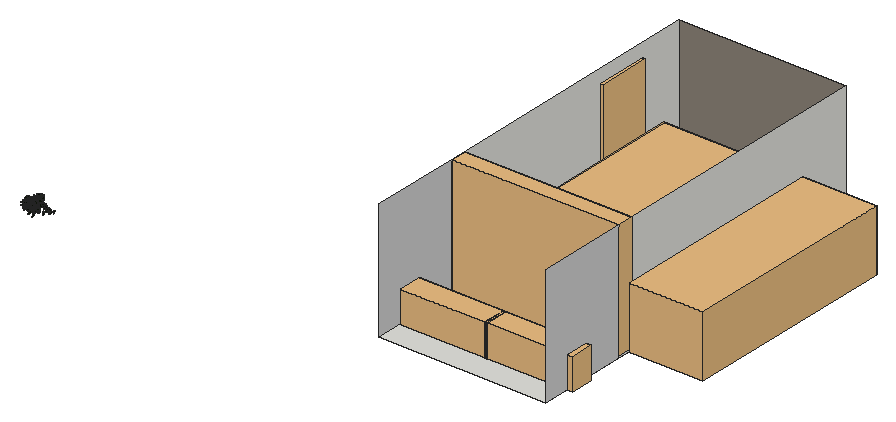
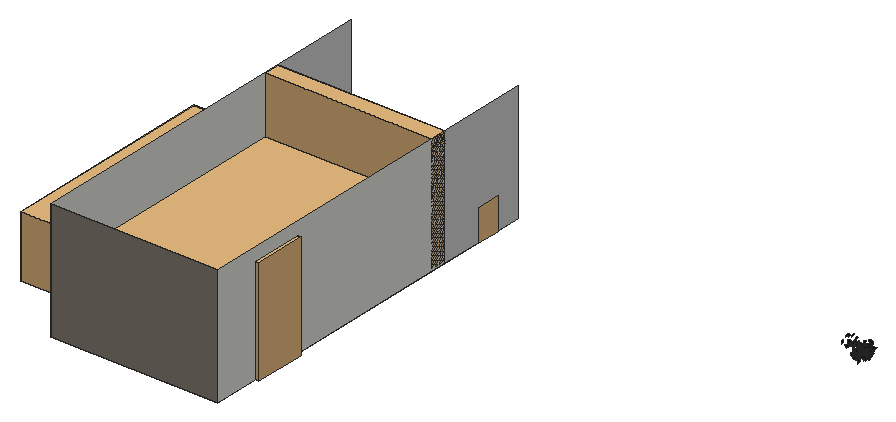
# SketchUp Ruby script. Lengths in inches.
U = 1.inch
M = Sketchup.active_model
def pt(a) = Geom::Point3d.new(a.map { |v| v * U })
def face(e, loops, mat)
  f = e.add_face(loops[0].map { |a| pt(a) })
  loops[1..].each { |l| e.add_face(l.map { |a| pt(a) }).erase! }
  f.material = f.back_material = mat if mat
  f
end
# faces: each face lists its corners as indices into pts; further lists are holes
def faces(e, pts, list, mat = nil) = list.each { |f| face(e, (f[0].is_a?(Array) ? f : [f]).map { |l| l.map { |i| pts[i] } }, mat) }
# xy, xz, yz: faces in a plane at the given z, y or x. An outline is a flat list of corners, or four numbers for a rectangle; further outlines are holes
def ring(l) = l.size == 4 ? [[l[0], l[1]], [l[2], l[1]], [l[2], l[3]], [l[0], l[3]]] : l.each_slice(2).to_a
def flat(e, list, mat, &to3) = list.each { |f| face(e, (f[0].is_a?(Array) ? f : [f]).map { |l| ring(l).map { |u, v| to3.(u, v) } }, mat) }
def xy(e, z, list, mat = nil) = flat(e, list, mat) { |x, y| [x, y, z] }
def xz(e, y, list, mat = nil) = flat(e, list, mat) { |x, z| [x, y, z] }
def yz(e, x, list, mat = nil) = flat(e, list, mat) { |y, z| [x, y, z] }
def lines(e, pts, list) = list.each { |a, b| e.add_line(pt(pts[a]), pt(pts[b])) }
# prism: a flat outline (further loops are holes) pulled along v
def prism(e, loops, v, mat = nil)
  f = face(e, loops, mat); d = Geom::Vector3d.new(v.map { |x| x * U })
  f.pushpull(f.normal.samedirection?(d) ? d.length : -d.length)
end
def box(e, o, s, mat = nil) = prism(e, [[o, [o[0] + s[0], o[1], o[2]], [o[0] + s[0], o[1] + s[1], o[2]], [o[0], o[1] + s[1], o[2]]]], [0, 0, s[2]], mat)
def at(x, y, z, deg = 0) = Geom::Transformation.translation(pt([x, y, z])) * Geom::Transformation.rotation(ORIGIN, Z_AXIS, deg.degrees)
def axes(o, x, y, z) = Geom::Transformation.new([*x, 0, *y, 0, *z, 0, *pt(o).to_a, 1])
def part(name) = M.definitions.add(name)
# library, detail: a bought-in or finely detailed component or shape, given as its bounding box
def library(name, o, s) = part(name).tap { |d| box(d.entities, o, s) }
def detail(e, o, s) = box(e.add_group.entities, o, s)
def put(e, d, t, mat = nil) = e.add_instance(d, t).tap { |i| i.material = mat if mat }
def group(e, t, mat = nil) = e.add_group.tap { |g| g.transformation = t; g.material = mat if mat }.entities
root = M.entities
M.materials.add("Concrete White 02 100cm").color = [209, 209, 209]
M.materials.add("Heather_Band").color = [140, 131, 120]
M.materials.add("efeu1").color = [18, 25, 13]
M.materials.add("efeu2").color = [43, 57, 29]
c1 = part("ivyleaf_9")
p = [[1.54,2.16,1.25],[1.36,2.04,1.19],[-0.21,0.99,0.68],[-0.71,1.11,0.82],[-0.85,0.86,0.67],[-0.8,0.17,0.21],
  [-0.9,-0.01,0.1],[-0.67,-0.16,-0.02],[-0.08,-0.08,-0.05],[-0.03,-0.6,-0.4],[0.65,-0.88,-0.66],[0.83,-0.6,-0.49],
  [1.29,-0.42,-0.43],[1.8125,-0.07,-0.26],[1.21,0.44,0.15]]
faces(c1.entities,p,[[0,1,2,3,4,5,6,7,8,9,10,11,12,13,14]],"efeu1")
c2 = part("ivyleaf_10")
p = [[0,0.5,-0.03],[-0.0625,2.02,-0.43],[-0.19,2.01,-0.46],[-0.54,1.05,-0.29],[-0.52,0.625,-0.18],[-0.83,0.76,-0.28],
  [-1.16,0.64,-0.33],[-1.15,0.33,-0.24],[-0.77,-0.39,0.02],[-0.3,-0.51,0.16],[0.04,-0.48,0.23],[-0.02,2.01,-0.4375],
  [-0.06,2.01,-0.43],[0.04,-0.49,0.23],[0.67,-0.49,0.14],[1.38,0.36,-0.2],[1.375,0.51,-0.24],[0.81,0.65,-0.19],
  [0.62,0.59,-0.15],[0.6,1.09,-0.28],[0.5,1.23,-0.31]]
faces(c2.entities,p,[[0,1,2,3,4,5,6,7,8,9,10],[11,12,0,13,14,15,16,17,18,19,20]],"efeu2")
c3 = library("Door 243 067",[-20.85,-3,0],[41.7,6,82.46])
c4 = library("Group\#39",[0,0,0],[56.8,25.91,35.15])
c5 = library("Group\#1",[0,0,0],[116.43,13.29,95.4])
c6 = library("BED_01",[-66.74,-61.37,0],[192.98,188.94,55.24])
xy(root,250.82,[[245.01,223.4375,337.3,430.75]])
xz(root,430.75,[[245.01,250.82,337.3,316.43]],"Heather_Band")
yz(root,245.01,[[273.83,250.82,430.75,316.43]])
yz(root,245.01,[[223.4375,250.82,273.83,316.43]],"Concrete White 02 100cm")
yz(root,337.3,[[273.83,250.82,430.75,316.43]])
yz(root,337.3,[[223.4375,250.82,273.83,316.43]],"Concrete White 02 100cm")
put(root,c1,axes([52.75,218.9375,252.16],[-0.28438,-0.06246,0.40648],[-0.38448,-0.135,-0.28974],[0.14595,-0.47736,0.02875]))
put(root,c2,axes([52.47,221.83,250.91],[0.22035,-0.44852,0.0165],[0.01087,-0.01304,-0.49971],[0.44869,0.22058,0.004]))
put(root,c1,axes([52.35,222.1,249.64],[0.06078,-0.49464,-0.04048],[-0.01,0.03955,-0.49833],[0.49619,0.06139,-0.00508]))
put(root,c1,axes([52.77,219.61,251.4],[-0.48579,-0.0978,0.06663],[-0.06405,-0.01942,-0.4955],[0.09951,-0.48996,0.00634]))
put(root,c1,axes([52.45,219.53,251.55],[-0.14793,-0.47101,-0.07914],[0.02295,0.07575,-0.4937],[0.47707,-0.14969,-0.00079]))
put(root,c2,axes([52.58,221.89,250.16],[-0.2895,-0.40666,-0.02848],[0.04763,0.00096,-0.49773],[0.40487,-0.2909,0.03818]))
put(root,c1,axes([52.25,219.97,249.66],[0.40442,-0.28864,0.05601],[0.0443,-0.03435,-0.49685],[0.29066,0.40683,-0.00221]))
put(root,c1,axes([52.9,220.99,250.11],[-0.39399,0.27889,0.13034],[-0.11839,0.05815,-0.48229],[-0.28417,-0.4109,0.02022]))
put(root,c1,axes([52.49,219.63,249.05],[0.00725,-0.4906,0.09621],[0.03502,-0.09548,-0.48955],[0.49872,0.01384,0.03297]))
put(root,c1,axes([52.47,222.04,248.69],[0.01453,-0.1929,0.46106],[0.08136,-0.45419,-0.19259],[0.49312,0.08062,0.01819]))
put(root,c2,axes([52.59,221.33,249.04],[0.49379,0.00255,0.07851],[0.07734,0.07153,-0.48877],[-0.01373,0.49485,0.07025]))
put(root,c1,axes([52.86,219.57,251.25],[-0.24859,-0.33217,0.27904],[-0.14378,-0.24034,-0.4142],[0.4093,-0.28618,0.02397]))
put(root,c1,axes([52.96,220.18,251.15],[-0.42268,0.22441,-0.14484],[0.12785,-0.06806,-0.47856],[-0.23451,-0.44159,0.00015]))
put(root,c1,axes([53.17,221.14,250.91],[-0.21403,0.03009,-0.45087],[-0.44991,0.03235,0.21573],[0.04216,0.49804,0.01323]))
put(root,c1,axes([53.04,221.73,250.3],[-0.47304,-0.11716,0.11183],[-0.09817,-0.06716,-0.48565],[0.12882,-0.48142,0.04054]))
put(root,c2,axes([52.75,220.1,251.3],[-0.45917,-0.03697,-0.19441],[0.19619,-0.02059,-0.45944],[0.02597,-0.49821,0.03341]))
put(root,c1,axes([52.93,221.27,251.05],[-0.22883,-0.32821,0.29986],[-0.12852,-0.27401,-0.39799],[0.42558,-0.25922,0.04105]))
put(root,c1,axes([52.65,219.89,251.02],[0.1245,-0.46683,0.12871],[0.03648,-0.12347,-0.48314],[0.48288,0.12969,0.00331]))
put(root,c1,axes([53.04,222.27,248.8125],[0.12734,-0.00585,-0.48348],[-0.39623,0.28527,-0.10781],[0.2771,0.41059,0.06801]))
put(root,c1,axes([53.23,217.88,250.86],[-0.24636,0.02606,0.43431],[-0.36929,-0.27643,-0.19289],[0.23007,-0.41582,0.15545]))
put(root,c2,axes([53.02,221.91,250.19],[-0.47246,-0.1627,-0.01754],[0.01571,0.00825,-0.49969],[0.16288,-0.47272,-0.00269]))
put(root,c1,axes([52.86,222.2,249.46],[0.37788,0.30295,0.1242],[0.08227,0.09573,-0.4838],[-0.31692,0.38608,0.02251]))
put(root,c1,axes([53.3125,221.74,248.83],[-0.40779,0.27712,0.08313],[-0.05838,0.06189,-0.49271],[-0.28337,-0.41155,-0.01812]))
put(root,c1,axes([52.89,221.26,253.7],[-0.03836,-0.49398,-0.06714],[-0.00426,0.06766,-0.49538],[0.49851,-0.03743,-0.0094]))
put(root,c2,axes([52.87,222.08,250.07],[-0.42151,0.00599,-0.26887],[0.25422,-0.15423,-0.40198],[-0.08775,-0.47558,0.12698]))
put(root,c2,axes([52.84,219.01,249.44],[0.34203,-0.22077,0.2903],[0.23517,-0.17069,-0.40689],[0.27876,0.41488,-0.01292]))
put(root,c2,axes([53.1,222.12,250.08],[-0.32219,0.36612,-0.11021],[-0.0064,-0.14926,-0.47716],[-0.3823,-0.30606,0.10086]))
put(root,c2,axes([53.18,221.82,251.35],[0.03306,-0.49395,0.07013],[-0.00013,-0.0703,-0.49503],[0.49891,0.03272,-0.00477]))
put(root,c1,axes([53.01,220.8125,253.05],[-0.02942,-0.48239,0.12821],[0.02307,-0.12961,-0.48236],[0.4986,-0.02246,0.02989]))
put(root,c1,axes([52.91,221.9,250.1],[0.47632,-0.15205,-0.00168],[0.00165,0.0107,-0.49988],[0.15205,0.4762,0.01069]))
put(root,c1,axes([53,221.34,251.11],[0.20913,-0.42782,-0.15243],[-0.06248,0.13912,-0.47617],[0.44985,0.21821,0.00472]))
put(root,c1,axes([53.14,221.62,251.15],[-0.11176,-0.00691,-0.4873],[0.42812,-0.24028,-0.09478],[-0.23286,-0.43843,0.05962]))
put(root,c1,axes([53.62,219.84,253.375],[-0.46338,0.17797,0.06008],[-0.05523,0.02377,-0.49637],[-0.17953,-0.46665,-0.00237]))
put(root,c1,axes([53.35,220.87,250.79],[-0.42199,0.01919,-0.2675],[0.26424,-0.05546,-0.42083],[-0.04582,-0.49654,0.03666]))
put(root,c1,axes([53.11,220.69,251.14],[0.47182,0.05572,0.15582],[0.12848,0.17335,-0.45104],[-0.10429,0.46567,0.14926]))
put(root,c1,axes([53.23,219.92,253.9],[0.00237,-0.49393,0.07766],[0.00693,-0.07762,-0.49389],[0.49995,0.00342,0.00648]))
put(root,c2,axes([53.61,221.19,251.73],[0.03108,0.20057,-0.45695],[-0.32674,-0.33788,-0.17053],[-0.37719,0.30921,0.11007]))
put(root,c1,axes([53.08,219.22,253.09],[0.39042,0.07898,0.30221],[0.28849,0.09432,-0.39734],[-0.11977,0.48463,0.02808]))
put(root,c1,axes([53.36,221.2,252.86],[0.43962,0.20913,-0.114],[-0.11606,-0.02088,-0.48589],[-0.20799,0.45368,0.03018]))
put(root,c1,axes([53.0625,221.86,250.78],[0.24519,-0.00115,0.43575],[0.43063,0.07708,-0.24211],[-0.06662,0.49402,0.03879]))
put(root,c1,axes([53.7,223.16,250.21],[-0.05184,0.029,0.49646],[-0.42819,-0.25646,-0.02973],[0.25292,-0.42824,0.05142]))
put(root,c1,axes([53.33,221.93,250.69],[0.12703,-0.45907,-0.15204],[-0.00561,0.15579,-0.47508],[0.48356,0.12241,0.03443]))
put(root,c1,axes([53.2,221.73,251.85],[0.41654,-0.26818,0.06767],[0.11093,0.04993,-0.48498],[0.25336,0.41903,0.10109]))
put(root,c2,axes([53.64,221.77,250.13],[-0.26707,-0.41433,0.08371],[-0.02681,-0.08222,-0.49246],[0.42185,-0.26753,0.0217]))
put(root,c1,axes([53.71,221.55,253.27],[-0.06186,0.49608,0.00893],[-0.00089,0.00889,-0.49992],[-0.49616,-0.06187,-0.00021]))
put(root,c1,axes([53.22,222.05,249.4],[0.44055,-0.15818,0.17578],[0.17732,-0.02491,-0.46684],[0.15644,0.47367,0.03415]))
put(root,c1,axes([53.4375,221.8,250.68],[-0.03058,-0.49693,-0.04607],[0.02021,0.04489,-0.49757],[0.49865,-0.0323,0.01734]))
put(root,c2,axes([53.66,223.28,252.39],[-0.30895,-0.39138,-0.03702],[0.02465,0.02771,-0.49862],[0.39236,-0.30992,0.00217]))
put(root,c1,axes([53.49,221.68,251.68],[-0.0509,-0.49733,0.00863],[0.01744,-0.01045,-0.49959],[0.4971,-0.05055,0.01841]))
put(root,c2,axes([53.65,226.8125,248.77],[-0.20297,0.45519,-0.04006],[0.01593,-0.03675,-0.49839],[-0.45667,-0.20359,0.00041]))
put(root,c1,axes([54.0625,220.31,252.92],[-0.20924,0.38084,0.24735],[-0.18772,0.17544,-0.42893],[-0.41349,-0.27237,0.06956]))
put(root,c1,axes([54.02,219.55,253.03],[-0.44745,0.2196,0.03952],[-0.03127,0.02597,-0.49835],[-0.22093,-0.44844,-0.00951]))
put(root,c1,axes([53.63,217.98,250.74],[-0.07469,-0.13513,0.47556],[-0.01867,-0.47985,-0.13928],[0.49404,-0.03856,0.06664]))
put(root,c1,axes([54.06,221.45,251.25],[-0.30102,0.33956,-0.20995],[0.04336,-0.23358,-0.43995],[-0.39687,-0.28308,0.11118]))
put(root,c2,axes([53.7,222.19,249.625],[0.02828,0.13737,0.47993],[0.12282,0.46401,-0.14005],[-0.48386,0.12581,-0.0075]))
put(root,c2,axes([53.95,223.46,248.875],[0.28588,-0.33686,-0.23409],[-0.1013,0.21852,-0.43816],[0.39751,0.29795,0.0567]))
put(root,c1,axes([53.71,221.75,250.87],[0.436,-0.21179,-0.12267],[-0.10792,0.05857,-0.48469],[0.21967,0.44913,0.00536]))
put(root,c1,axes([53.91,226.61,249.14],[0.39293,-0.06499,-0.30229],[-0.28177,0.12602,-0.39335],[0.12732,0.47947,0.06241]))
put(root,c2,axes([54.08,223.76,251.27],[-0.42306,-0.2561,0.07369],[-0.0609,-0.04169,-0.49452],[0.25944,-0.42741,0.00409]))
put(root,c1,axes([53.93,221.5,251.99],[-0.17719,-0.46752,0.00533],[0.05162,-0.02523,-0.49669],[0.46469,-0.17547,0.05721]))
put(root,c2,axes([54.08,223.6,252.47],[0.48661,-0.06777,-0.09282],[-0.09017,0.02525,-0.49115],[0.07126,0.49474,0.01235]))
put(root,c2,axes([54.18,221.74,252.19],[-0.26259,-0.4252,0.01605],[-0.01389,-0.01028,-0.4997],[0.42527,-0.26287,-0.00641]))
put(root,c1,axes([54.09,226.57,249.29],[0.40254,0.25953,-0.14356],[-0.12182,-0.07598,-0.47894],[-0.27041,0.42056,0.00206]))
put(root,c1,axes([54.17,223.61,249.3],[-0.37777,-0.31991,-0.07035],[0.05735,0.04113,-0.49499],[0.32249,-0.38205,0.00562]))
put(root,c2,axes([54.1,222.09,248.93],[-0.34219,-0.32394,-0.16725],[0.13833,0.09685,-0.47062],[0.3373,-0.36835,0.02334]))
put(root,c1,axes([54.17,224.43,250.21],[-0.27482,-0.41237,0.06653],[-0.01724,-0.06837,-0.495],[0.41734,-0.27437,0.02336]))
put(root,c2,axes([54.2,222.02,251.38],[0.09571,-0.47445,0.12545],[0.00788,-0.12631,-0.48372],[0.49069,0.09457,-0.01671]))
put(root,c1,axes([53.96,221.69,252.02],[-0.01572,-0.46117,0.19256],[0.10401,-0.19145,-0.45003],[0.48881,0.02591,0.10195]))
put(root,c1,axes([53.95,218.96,249.51],[-0.08055,0.10808,0.48149],[0.23184,-0.42237,0.1336],[0.43562,0.24478,0.01793]))
put(root,c1,axes([54.44,222.38,249.05],[-0.4859,-0.11362,0.03144],[-0.02515,-0.03037,-0.49844],[0.11518,-0.48597,0.0238]))
put(root,c1,axes([54.28,223.22,250.33],[-0.35521,-0.34561,-0.06618],[0.06821,0.02462,-0.49471],[0.34521,-0.36049,0.02966]))
put(root,c1,axes([54.43,226.46,252.76],[-0.01985,-0.04222,-0.49782],[0.02303,-0.49776,0.0413],[-0.49907,-0.02129,0.02171]))
put(root,c1,axes([54.11,220.66,253.09],[0.2235,-0.36668,-0.25611],[-0.07271,0.25271,-0.42527],[0.44132,0.22734,0.05964]))
put(root,c1,axes([54.61,221.07,252.17],[-0.45886,0.19861,-0.0012],[0.00081,-0.00115,-0.5],[-0.19861,-0.45886,0.00074]))
put(root,c1,axes([54.57,226.25,253.07],[-0.14044,0.47781,0.04439],[-0.00631,0.04441,-0.49798],[-0.47983,-0.14043,-0.00645]))
put(root,c2,axes([54.375,221.91,251.91],[0.16597,-0.46469,0.08071],[0.03716,-0.07241,-0.49333],[0.47018,0.16976,0.0105]))
put(root,c1,axes([54.48,226.7,249.93],[-0.46911,-0.12881,-0.1155],[0.11206,0.02809,-0.48647],[0.13181,-0.48231,0.00251]))
put(root,c1,axes([54.43,219.68,250.55],[-0.323,-0.34887,0.15479],[0.00172,-0.20411,-0.45644],[0.38167,-0.29433,0.13306]))
put(root,c1,axes([54.18,221.72,248.85],[0.33326,-0.36581,-0.07155],[-0.01152,0.08583,-0.49244],[0.37257,0.32987,0.04878]))
put(root,c1,axes([54.21,222.18,249.29],[0.23019,-0.43398,-0.09313],[-0.00057,0.10462,-0.48893],[0.44386,0.2252,0.04767]))
put(root,c1,axes([54.65,221.94,250.25],[0.00155,0.46759,-0.17709],[-0.07961,-0.1746,-0.46171],[-0.49362,0.02963,0.07391]))
put(root,c2,axes([54.43,226.8,250.23],[-0.05243,0.49536,0.04318],[-0.00543,0.04285,-0.49813],[-0.49721,-0.05271,0.00089]))
put(root,c2,axes([54.42,221.92,249.09],[0.11517,0.48395,0.05029],[0.0051,0.05048,-0.49742],[-0.48653,0.11509,0.00669]))
put(root,c2,axes([54.54,222.05,249.9],[0.34693,0.30208,-0.19593],[-0.14547,-0.13129,-0.46],[-0.32936,0.37618,-0.00321]))
put(root,c1,axes([54.57,223.99,253.4],[0.40196,0.13977,-0.26248],[-0.2681,-0.02061,-0.42154],[-0.12866,0.47962,0.05838]))
put(root,c2,axes([54.51,226.34,253.14],[-0.16663,0.4714,-0.00362],[0.00144,-0.00334,-0.49999],[-0.47142,-0.16664,-0.00025]))
put(root,c1,axes([54.47,221.89,251.72],[-0.21044,-0.43038,-0.14314],[0.07031,0.12493,-0.47901],[0.44807,-0.22174,0.00794]))
put(root,c2,axes([54.21,222.23,251.32],[-0.11351,-0.45159,0.18215],[0.48694,-0.10466,0.04398],[-0.0016,0.18738,0.46356]))
put(root,c1,axes([54.48,221.46,252.91],[0.36962,0.33456,0.03805],[0.02528,0.02877,-0.49853],[-0.33577,0.37046,0.00435]))
put(root,c2,axes([54.64,221.83,252.48],[-0.1201,-0.48432,0.03172],[-0.00254,-0.03205,-0.49897],[0.48536,-0.12001,0.00524]))
put(root,c1,axes([54.32,222.26,252.12],[-0.12492,-0.43588,0.21072],[0.34952,-0.23177,-0.27224],[0.33501,0.07928,0.3626]))
put(root,c1,axes([54.89,217.76,252.44],[-0.34021,-0.35862,-0.07514],[-0.04971,-0.05641,0.49431],[-0.36302,0.34382,0.00273]))
put(root,c2,axes([54.59,221.64,252.81],[-0.45753,0.19558,-0.0491],[0.04316,-0.02393,-0.49756],[-0.19698,-0.45954,0.00501]))
put(root,c1,axes([54.6875,220.9,251.34],[-0.42894,-0.24588,-0.07454],[0.06969,0.02827,-0.49431],[0.2473,-0.43445,0.01002]))
put(root,c2,axes([54.58,223.97,253.375],[0.24341,0.42264,-0.11014],[-0.05743,-0.09403,-0.48771],[-0.43296,0.25007,0.00277]))
put(root,c1,axes([54.32,221.66,252.98],[0.36258,-0.34378,-0.01872],[0.05151,0.08105,-0.49069],[0.34041,0.3539,0.09419]))
put(root,c1,axes([54.42,222.01,251.7],[0.13917,-0.46899,-0.10333],[-0.00256,0.10685,-0.48844],[0.48023,0.13648,0.02734]))
put(root,c1,axes([54.375,222.15,251.92],[-0.11325,-0.46147,-0.15564],[0.48695,-0.10483,-0.04352],[0.00754,-0.16143,0.47316]))
put(root,c1,axes([55,221.35,249.22],[-0.41622,-0.02346,0.27606],[-0.26865,-0.0876,-0.41249],[0.06772,-0.49171,0.06031]))
put(root,c1,axes([54.57,221.7,252.46],[0.41939,-0.06578,-0.26418],[-0.22626,0.18562,-0.40541],[0.1514,0.45959,0.12593]))
put(root,c1,axes([54.82,221.46,253.54],[-0.01212,0.45455,-0.20793],[-0.00724,-0.20813,-0.45457],[-0.4998,-0.00801,0.01163]))
put(root,c2,axes([54.51,221.9,252.06],[0.42597,-0.20332,0.16496],[0.17649,-0.0097,-0.46771],[0.19339,0.45669,0.06351]))
put(root,c1,axes([54.5,220.99,249.58],[0.01551,-0.49417,-0.07456],[0.01724,0.07508,-0.49403],[0.49946,0.01275,0.01936]))
put(root,c1,axes([54.56,219.8,248.74],[0.29194,0.33904,0.22321],[0.14514,0.16958,-0.44741],[-0.37908,0.32603,0.0006]))
put(root,c2,axes([54.63,222.03,249.33],[0.33664,-0.34565,0.13115],[0.1178,-0.06785,-0.48117],[0.35042,0.35486,0.03576]))
put(root,c2,axes([54.68,221.86,252.08],[0.37278,-0.33296,-0.01327],[0.09863,0.12927,-0.47282],[0.31829,0.3499,0.16206]))
put(root,c2,axes([54.8125,226.79,251.31],[-0.49903,-0.02674,-0.0161],[0.01872,-0.05013,-0.49713],[0.02497,-0.49676,0.05103]))
put(root,c1,axes([54.56,221.74,252.02],[0.10748,-0.46924,0.13515],[0.07761,-0.12021,-0.47909],[0.48211,0.12396,0.04699]))
put(root,c1,axes([54.4,216.96,253.18],[0.32576,-0.15351,0.34686],[0.31987,-0.13455,-0.35997],[0.20386,0.45643,0.01055]))
put(root,c2,axes([54.78,221.06,250.6],[-0.34752,-0.30717,-0.18675],[0.14886,0.11346,-0.46365],[0.32721,-0.37785,0.01259]))
put(root,c2,axes([54.52,222.76,250.21],[0.32316,-0.37906,-0.04336],[0.38151,0.32165,0.03143],[0.00406,-0.0534,0.49712]))
put(root,c1,axes([54.54,219.68,253.49],[0.46655,-0.12864,0.12565],[0.13673,0.02688,-0.48019],[0.11679,0.48242,0.06026]))
put(root,c2,axes([54.94,221.76,248.7],[-0.32203,0.38227,0.01304],[-0.01245,0.00657,-0.4998],[-0.38229,-0.32222,0.00529]))
put(root,c2,axes([54.81,222.02,250.8],[-0.27651,0.25262,-0.33125],[0.20675,-0.26194,-0.37235],[-0.36166,-0.34289,0.0404]))
put(root,c2,axes([55.06,221.77,252.7],[0.42161,-0.18119,-0.19855],[-0.13561,0.17551,-0.44812],[0.23208,0.4317,0.09885]))
put(root,c2,axes([54.67,222.27,250.96],[0.19082,-0.45081,0.10179],[0.43885,0.14221,-0.19284],[0.14492,0.16294,0.44995]))
put(root,c1,axes([55.14,221.48,249.05],[-0.41261,-0.22889,0.16542],[-0.04443,-0.23661,-0.43823],[0.27889,-0.37633,0.17491]))
put(root,c1,axes([55.2,226.28,253.45],[-0.01458,0.47731,-0.14819],[-0.01503,-0.14861,-0.47717],[-0.49956,-0.00946,0.01869]))
put(root,c1,axes([55.23,222.61,251.12],[-0.25635,0.40485,-0.14276],[0.08814,-0.1131,-0.479],[-0.42013,-0.27075,-0.01338]))
put(root,c1,axes([55.17,217.58,252.51],[-0.22789,-0.33995,0.28722],[-0.17114,-0.23094,-0.40912],[0.41083,-0.28478,-0.01111]))
put(root,c1,axes([54.9,221.54,251.4375],[0.46972,0.16965,0.02422],[0.02352,0.00618,-0.49941],[-0.16975,0.4703,-0.00217]))
put(root,c1,axes([55.01,221.97,249.86],[0.01223,-0.49984,0.00343],[0.00009,-0.00343,-0.49999],[0.49985,0.01223,0.00001]))
put(root,c2,axes([55.23,221.625,252.79],[-0.3719,0.33196,0.03866],[-0.02756,0.02718,-0.4985],[-0.33307,-0.37291,-0.00192]))
put(root,c1,axes([55.03,221.72,253.15],[-0.23427,0.08468,0.43353],[0.40658,-0.15046,0.2491],[0.17264,0.46925,0.00164]))
put(root,c1,axes([55.48,221.04,250.3],[0.13477,0.41137,-0.25022],[-0.26714,-0.1523,-0.39426],[-0.4006,0.23995,0.17873]))
put(root,c2,axes([55.26,225.02,248.85],[-0.00138,-0.07146,-0.49486],[-0.08026,-0.48842,0.07076],[-0.49351,0.07963,-0.01012]))
put(root,c2,axes([55.37,222.27,250.42],[-0.16015,-0.47362,0.00616],[-0.00797,-0.0038,-0.49992],[0.47359,-0.16022,-0.00633]))
put(root,c1,axes([55.39,226.66,251.53],[-0.34704,0.16147,-0.3217],[0.25519,-0.20478,-0.37808],[-0.25385,-0.42661,0.05972]))
put(root,c1,axes([54.97,220.17,253.0625],[0.34503,0.18881,-0.30872],[0.2041,0.2507,0.38144],[0.29883,-0.38923,0.09592]))
put(root,c2,axes([55.01,222,248.37],[0.2788,-0.05067,-0.41195],[0.41288,-0.01688,0.2815],[-0.04243,-0.49714,0.03243]))
put(root,c1,axes([55.33,221.9375,250.34],[-0.2689,-0.41465,-0.07589],[0.05319,0.05591,-0.49401],[0.41817,-0.27375,0.01404]))
put(root,c1,axes([55.22,217.02,251.37],[0.01617,-0.1497,0.47679],[0.02067,-0.47643,-0.15029],[0.49931,0.02457,-0.00922]))
put(root,c1,axes([55.64,220.4,253.35],[-0.48129,0.13544,-0.00397],[0.00379,-0.00121,-0.49998],[-0.13544,-0.48131,0.00014]))
put(root,c2,axes([55.34,221.95,248.85],[0.33554,-0.35905,0.09216],[0.09565,-0.03623,-0.48943],[0.35814,0.34607,0.04437]))
put(root,c1,axes([55.56,221.91,249.07],[0.03695,0.49578,-0.05325],[-0.00286,-0.05319,-0.49715],[-0.49862,0.03705,-0.00109]))
put(root,c2,axes([55.3,221.39,251.94],[-0.42017,-0.15359,-0.22331],[0.25284,-0.07372,-0.42502],[0.09763,-0.47008,0.13962]))
put(root,c2,axes([55.49,222.01,250.9],[0.1045,0.37554,-0.31313],[-0.10479,-0.29556,-0.38944],[-0.4776,0.14702,0.01693]))
put(root,c2,axes([55.41,219.73,251.05],[0.34507,-0.35255,0.08147],[0.09585,-0.0195,-0.49034],[0.34891,0.35402,0.05413]))
put(root,c2,axes([55.58,225.0625,250.8125],[-0.06016,-0.45601,0.19604],[-0.04199,-0.19209,-0.45972],[0.49459,-0.07178,-0.01519]))
put(root,c1,axes([55.57,222.6,249.53],[0.10431,0.25651,0.41632],[0.09389,0.40726,-0.27445],[-0.4799,0.13544,0.0368]))
put(root,c1,axes([55.79,221.6,251.4],[-0.25814,0.42744,-0.0256],[0.01485,-0.02094,-0.49934],[-0.42795,-0.25856,-0.00188]))
put(root,c1,axes([55.27,221.21,253.45],[0.44818,-0.14417,0.16838],[0.19102,0.05851,-0.45835],[0.11246,0.47517,0.10752]))
put(root,c1,axes([55.7,221.93,251.12],[0.29028,0.40688,-0.01357],[-0.00824,-0.01078,-0.49982],[-0.40702,0.2904,0.00045]))
put(root,c1,axes([56.06,224.94,249.48],[-0.22167,0.36344,0.26224],[-0.14834,0.21658,-0.42555],[-0.42291,-0.26647,0.01181]))
put(root,c1,axes([55.63,221.24,253.7],[0.00532,-0.49823,-0.04175],[-0.00176,0.04173,-0.49825],[0.49997,0.00544,-0.00131]))
put(root,c1,axes([56.15,221.4375,253.16],[-0.17463,0.24543,0.39909],[-0.24658,0.314,-0.301],[-0.39838,-0.30194,0.01137]))
put(root,c1,axes([55.95,221.58,253.01],[0.02658,0.49397,-0.07269],[0.0122,-0.07342,-0.49443],[-0.49914,0.02451,-0.01596]))
put(root,c1,axes([55.73,220.4,248.98],[-0.2721,0.0287,-0.4185],[0.4093,-0.09108,-0.27236],[-0.09186,-0.4908,0.02607]))
put(root,c1,axes([56.03,217.7,250.8125],[-0.03117,0.25162,0.43095],[-0.03399,0.42971,-0.25336],[-0.49787,-0.04509,-0.00969]))
put(root,c1,axes([56.1,221.58,253.57],[-0.49337,0.07759,-0.02387],[0.01258,-0.07212,-0.49461],[-0.08019,-0.48865,0.06921]))
put(root,c1,axes([55.49,222.01,251.09],[0.32797,-0.27843,0.25478],[0.20396,-0.15324,-0.43002],[0.31755,0.386,0.01306]))
put(root,c1,axes([56.02,226.59,251.2],[-0.45968,-0.19593,-0.01764],[0.01598,0.00749,-0.49969],[0.19607,-0.45995,-0.00063]))
put(root,c2,axes([55.84,226.97,252.16],[-0.2327,-0.37587,-0.23361],[0.1647,0.17142,-0.43987],[0.41076,-0.28166,0.04403]))
put(root,c1,axes([55.82,221.81,253.47],[-0.14158,-0.4773,0.04631],[0.00352,-0.04932,-0.49755],[0.47952,-0.14056,0.01733]))
put(root,c1,axes([56.01,216.63,253.88],[0.34574,0.04085,-0.35888],[-0.35364,-0.06285,-0.34784],[-0.07353,0.49435,-0.01457]))
put(root,c2,axes([55.98,221.88,249.55],[0.1708,-0.45131,-0.13093],[-0.01514,0.13395,-0.48148],[0.46968,0.16844,0.03209]))
put(root,c2,axes([56.07,221.0625,249.88],[-0.23591,-0.38606,0.21284],[-0.08143,-0.19909,-0.45137],[0.43326,-0.24763,0.03106]))
put(root,c1,axes([55.68,221.99,250.93],[0.32762,-0.36311,0.10402],[0.05976,-0.08613,-0.48889],[0.37296,0.33277,-0.01303]))
put(root,c1,axes([55.92,221.94,251.39],[-0.02216,-0.46069,0.19306],[-0.02126,-0.19221,-0.46109],[0.49906,-0.02865,-0.01107]))
put(root,c1,axes([55.95,221.22,251.99],[-0.05456,-0.46229,0.1825],[0.03145,-0.18644,-0.46287],[0.49602,-0.03903,0.04943]))
put(root,c1,axes([56.27,220.29,249.42],[0.21192,-0.03511,-0.45151],[-0.44145,0.09521,-0.2146],[0.10105,0.48959,0.00935]))
put(root,c1,axes([56.375,220.9375,253.56],[-0.49449,-0.03572,0.06486],[-0.06467,-0.00498,-0.49578],[0.03607,-0.4987,0.00031]))
put(root,c2,axes([56.22,221.28,250.97],[-0.48547,-0.11802,0.01976],[-0.02019,-0.00059,-0.49959],[0.11795,-0.48587,-0.00419]))
put(root,c1,axes([56.13,221.6875,252.72],[-0.13353,-0.10998,0.46912],[-0.00592,-0.48639,-0.11572],[0.4818,-0.03646,0.12859]))
put(root,c1,axes([56.01,217.82,250.17],[0.12635,-0.48194,0.04206],[0.01774,-0.03882,-0.49817],[0.48345,0.12738,0.00729]))
put(root,c1,axes([56.43,226.71,252.67],[-0.11513,0.35673,-0.33089],[-0.00618,-0.34107,-0.36555],[-0.48652,-0.08008,0.08295]))
put(root,c1,axes([56.39,226.57,253.27],[-0.48308,-0.11717,-0.05393],[0.07657,-0.09223,-0.48542],[0.10381,-0.47725,0.10705]))
put(root,c2,axes([56.11,221.625,251.88],[0.15452,-0.36022,0.31042],[0.30763,-0.17317,-0.35408],[0.36261,0.30042,0.16811]))
put(root,c1,axes([56.52,224.99,249.85],[0.1666,0.41449,-0.22459],[-0.19333,-0.15718,-0.43349],[-0.42996,0.23128,0.1079]))
put(root,c1,axes([56.15,220.18,250.39],[0.04307,-0.05035,-0.49559],[0.26419,0.42402,-0.02012],[0.42231,-0.26013,0.06313]))
put(root,c1,axes([56.32,224.875,248.99],[0.21517,-0.30983,-0.32819],[-0.08696,0.3283,-0.36695],[0.44288,0.21499,0.0874]))
put(root,c2,axes([56.41,226.74,253.18],[0.22719,0.43107,0.1121],[0.03488,0.10823,-0.4869],[-0.44404,0.22905,0.0191]))
put(root,c1,axes([56.83,223.42,249.36],[-0.12117,0.36539,0.31907],[-0.20538,0.2593,-0.37494],[-0.43947,-0.22193,0.08725]))
put(root,c1,axes([56.72,226.32,251.96],[0.22586,-0.12047,0.4295],[-0.36794,0.22188,0.25572],[-0.25221,-0.43158,0.01158]))
put(root,c1,axes([56.46,219.57,251.73],[-0.29129,0.0651,-0.40114],[0.38524,-0.11291,-0.29807],[-0.12939,-0.48272,0.01562]))
put(root,c2,axes([56.6,226.56,253.08],[0.23157,0.40575,-0.17816],[-0.08806,-0.15487,-0.46718],[-0.4343,0.24775,-0.00027]))
put(root,c1,axes([56.81,219.78,251.48],[0.14501,0.29043,-0.3803],[-0.17079,-0.33979,-0.32461],[-0.44699,0.22405,0.00066]))
put(root,c2,axes([56.7,221.26,252.98],[-0.47118,0.13743,-0.09539],[0.07798,-0.0718,-0.48863],[-0.148,-0.47535,0.04623]))
put(root,c1,axes([56.97,217.61,248.7],[0.08862,0.04611,0.48992],[-0.46306,-0.16062,0.09888],[0.1665,-0.47125,0.01424]))
put(root,c2,axes([56.58,220.14,248.83],[-0.2132,0.17216,-0.41822],[0.24044,-0.34846,-0.26602],[-0.38306,-0.31454,0.06579]))
put(root,c1,axes([56.67,221.11,253.17],[-0.07902,-0.48811,-0.0742],[0.01086,0.07341,-0.49446],[0.4936,-0.07975,-0.001]))
put(root,c1,axes([56.75,221.73,251.78],[-0.17311,-0.45781,-0.10218],[0.03523,0.09592,-0.48945],[0.46775,-0.17666,-0.00095]))
put(root,c1,axes([56.66,226.81,252.16],[0.20664,-0.4239,-0.16616],[-0.0584,0.15629,-0.47134],[0.45154,0.2142,0.01507]))
put(root,c1,axes([56.78,221.76,250.57],[0.10762,-0.48582,-0.04892],[-0.00839,0.04825,-0.4976],[0.48821,0.10793,0.00224]))
put(root,c1,axes([57.04,220.71,253.09],[-0.21659,-0.23201,0.38634],[-0.13508,-0.37551,-0.30123],[0.42993,-0.23486,0.09998]))
put(root,c1,axes([57.3,221.27,253.61],[-0.3168,0.38683,0.00051],[0.01228,0.01072,-0.49973],[-0.38664,-0.31662,-0.0163]))
put(root,c2,axes([57.06,226.82,253.3],[-0.03934,0.08802,-0.49062],[-0.01356,-0.49215,-0.08721],[-0.49827,0.00644,0.04111]))
put(root,c1,axes([56.95,219.22,249.84],[0.01569,-0.42052,-0.27003],[0.0352,0.27043,-0.41908],[0.49851,-0.00586,0.03809]))
put(root,c1,axes([57.29,220.59,251.05],[-0.44015,-0.23707,-0.0083],[0.0071,0.00432,-0.49993],[0.23711,-0.4402,-0.00043]))
put(root,c1,axes([57.14,226.39,252.5625],[-0.26168,-0.42283,0.05236],[0.03137,-0.0804,-0.4925],[0.4249,-0.25446,0.0686]))
put(root,c1,axes([56.99,220.875,249.38],[-0.05324,-0.05814,0.49375],[0.14091,-0.47797,-0.04109],[0.47677,0.13477,0.06728]))
put(root,c1,axes([56.91,219.15,253.66],[0.13731,-0.33219,0.34756],[0.1687,-0.30518,-0.35833],[0.45021,0.21567,0.02827]))
put(root,c1,axes([57,221.15,251.95],[0.37133,-0.3302,-0.05555],[-0.04015,0.03844,-0.4969],[0.33242,0.37348,0.00203]))
put(root,c1,axes([57.41,221.7,251.25],[-0.04569,0.49791,-0.00048],[-0.00007,-0.00049,-0.5],[-0.49791,-0.04569,0.00012]))
put(root,c2,axes([57.2,223.58,249.77],[0.46121,-0.18934,0.03791],[0.03685,-0.01007,-0.49854],[0.18955,0.46266,0.00467]))
put(root,c1,axes([56.99,221.82,252.96],[0.2134,-0.4379,0.11272],[0.05535,-0.09841,-0.48709],[0.44877,0.22036,0.00648]))
put(root,c2,axes([57.25,225.03,250.74],[0.29494,0.39684,-0.07437],[-0.05171,-0.05421,-0.49436],[-0.40042,0.2993,0.00906]))
put(root,c1,axes([57.78,221.5,249.97],[-0.25534,0.31275,0.29494],[-0.26863,0.15174,-0.39347],[-0.33562,-0.35939,0.09053]))
put(root,c1,axes([57.7,221.78,251.29],[-0.49379,-0.07783,0.01061],[-0.01061,-0.00078,-0.49989],[0.07783,-0.49391,-0.00088]))
put(root,c1,axes([57.39,221.7,251.05],[-0.03538,-0.49822,0.02283],[-0.01417,-0.02188,-0.49932],[0.49855,-0.03598,-0.01257]))
put(root,c1,axes([57.79,221.15,252.84],[-0.03914,0.33011,0.37349],[-0.09952,0.36192,-0.33032],[-0.48843,-0.1002,0.03738]))
put(root,c1,axes([57.45,221.14,253.09],[-0.04786,-0.43415,0.24336],[0.00366,-0.24479,-0.43597],[0.49769,-0.03995,0.02661]))
put(root,c1,axes([57.55,219.91,252.16],[0.32037,-0.21204,-0.32001],[-0.27065,0.17083,-0.38414],[0.27224,0.41935,-0.00532]))
put(root,c1,axes([57.64,221.5625,252.76],[-0.31037,-0.33981,-0.19544],[0.13215,0.14399,-0.46022],[0.36906,-0.33733,0.00043]))
put(root,c1,axes([57.35,221.75,253.27],[0.21427,-0.28097,0.35376],[0.21375,-0.28188,-0.35335],[0.398,0.30265,-0.00068]))
put(root,c2,axes([57.84,222.36,252.79],[0.4195,-0.16516,-0.2162],[-0.17266,0.14546,-0.44613],[0.21026,0.44896,0.06501]))
put(root,c1,axes([57.625,225.0625,248.83],[0.43166,-0.2251,0.114],[0.09617,-0.06208,-0.48672],[0.23328,0.44213,-0.0103]))
put(root,c1,axes([58.14,219.68,249.3],[0.0379,0.49213,-0.07982],[-0.00842,-0.07941,-0.49358],[-0.49849,0.03876,0.00227]))
put(root,c2,axes([57.91,221.98,253.51],[0.48259,-0.11346,0.06504],[0.07872,0.05343,-0.49087],[0.10443,0.48402,0.06943]))
put(root,c1,axes([57.94,220.16,252.33],[0.24439,-0.42813,-0.08353],[-0.02187,0.0836,-0.49248],[0.43566,0.24437,0.02213]))
put(root,c1,axes([58.31,219.53,249.42],[-0.31469,-0.02449,-0.38778],[0.38705,0.02412,-0.31562],[0.03416,-0.49882,0.00378]))
put(root,c1,axes([58.67,221.57,252.88],[0.01384,0.45123,-0.21494],[-0.08777,-0.20949,-0.44543],[-0.49204,0.05006,0.07341]))
put(root,c1,axes([58.45,221.34,250.52],[-0.12706,-0.37709,0.30276],[-0.08476,-0.29082,-0.39779],[0.4761,-0.15241,0.00998]))
put(root,c1,axes([58.78,221.53,252.92],[0.14801,0.01502,0.47736],[-0.47531,-0.0442,0.14876],[0.04666,-0.49782,0.00119]))
put(root,c1,axes([58.74,217.28,251.03],[0.26269,-0.01806,-0.42505],[-0.40181,0.15363,-0.25485],[0.13981,0.47547,0.0662]))
put(root,c1,axes([58.95,221.5,253.08],[-0.05197,0.49727,-0.00462],[0.00008,-0.00463,-0.49998],[-0.49729,-0.05197,0.0004]))
put(root,c1,axes([58.59,220.57,252.44],[-0.09931,-0.03043,0.48909],[0.48779,0.04161,0.10163],[-0.04689,0.49734,0.02143]))
put(root,c1,axes([58.74,221.53,252.85],[0.05983,-0.4964,0.00247],[0.00194,-0.00225,-0.49999],[0.4964,0.05984,0.00166]))
put(root,c1,axes([59.1,225.6,249.87],[-0.34418,0.22153,-0.28717],[0.24526,-0.14949,-0.40927],[-0.26719,-0.42258,-0.00577]))
put(root,c1,axes([59.28,221.2,248.95],[-0.14072,-0.14185,0.45834],[-0.30311,-0.34397,-0.19952],[0.37191,-0.33401,0.01081]))
put(root,c1,axes([59,221.34,250.64],[0.14419,-0.47756,-0.03392],[-0.0133,0.03141,-0.49883],[0.47857,0.14476,-0.00365]))
put(root,c1,axes([59.06,220.92,250],[0.00452,-0.4972,-0.05265],[-0.00195,0.05264,-0.49722],[0.49998,0.0047,-0.00146]))
put(root,c1,axes([59.46,220.54,248.6],[-0.49508,0.05852,0.03831],[0.03776,-0.00683,0.49853],[0.05887,0.49652,0.00234]))
put(root,c1,axes([59.4375,221.54,253.17],[0.26036,0.41318,0.10723],[0.03576,0.10405,-0.48774],[-0.42536,0.26165,0.02463]))
put(root,c1,axes([59.39,216.8125,248.3125],[0.11583,0.2867,0.39292],[-0.15268,-0.36206,0.30919],[0.46181,-0.19161,0.00367]))
put(root,c1,axes([59.92,220.73,252.4],[0.10382,0.12955,0.47163],[-0.31864,-0.34787,0.16569],[0.37107,-0.33496,0.01033]))
put(root,c1,axes([59.73,221.42,253.99],[-0.11505,-0.3534,-0.33447],[0.11872,0.31292,-0.37146],[0.47188,-0.16489,0.01191]))
put(root,c1,axes([60.51,219.7,249.625],[-0.29214,0.38369,0.13205],[-0.08384,0.10212,-0.48223],[-0.39702,-0.30389,0.00467]))
put(root,c1,axes([61.28,221.29,252.95],[0.18888,-0.12931,-0.44453],[-0.2294,0.39088,-0.21117],[0.40212,0.28372,0.08833]))
put(root,c1,axes([61.52,220.99,253.2],[-0.39125,-0.26624,0.16138],[-0.07738,-0.16789,-0.46457],[0.30156,-0.3885,0.09017]))
put(root,c1,axes([62.1,218.85,253.48],[-0.1281,-0.34033,0.34317],[-0.12432,-0.31987,-0.36363],[0.46705,-0.17849,-0.00267]))
put(root,c1,axes([62.49,221.69,251.82],[0.27553,-0.36583,-0.20062],[-0.0841,0.18679,-0.45611],[0.40867,0.28509,0.0414]))
put(root,c1,axes([62.89,221.75,251.91],[-0.39692,0.00824,-0.30395],[0.30312,-0.02855,-0.39662],[-0.02389,-0.49912,0.01767]))
put(root,c1,axes([63.25,219.25,249.95],[-0.02947,-0.30426,0.39568],[0.02874,-0.39674,-0.30294],[0.4983,0.00489,0.04087]))
put(root,c1,axes([64.24,220.77,251.12],[-0.32095,-0.21355,0.31842],[-0.27509,-0.16099,-0.38524],[0.26706,-0.42247,-0.01415]))
put(root,c1,axes([64.37,220.37,252.54],[0.19754,0.23305,-0.39581],[-0.30195,-0.25879,-0.30307],[-0.34612,0.35877,0.03849]))
put(root,c1,axes([64.56,218.08,253.83],[-0.04812,-0.37237,0.33019],[0.00616,-0.33215,-0.37368],[0.49764,-0.0319,0.03655]))
put(root,c1,axes([64.8,221.19,249.79],[0.06002,-0.09788,0.48664],[0.48456,-0.0948,-0.07883],[0.1077,0.48107,0.08347]))
put(root,c1,axes([66.64,217.95,253.45],[0.07017,-0.02685,-0.49432],[0.42566,0.25818,0.04641],[0.25276,-0.42734,0.05909]))
put(root,c1,axes([67.2,218.63,253.34],[0.12484,-0.43372,0.21517],[0.05072,-0.20927,-0.45126],[0.4815,0.1345,-0.00825]))
put(root,c1,axes([67.53,220.96,251.43],[0.10893,0.00395,-0.48797],[-0.37385,0.32202,-0.08085],[0.31364,0.38248,0.07311]))
put(root,c3,axes([245.01,390.39,250.82],[0,0.68565,0],[-0.71,0,0],[0,0,0.71]))
put(root,c4,axes([244.62,237.87,250.76],[0.855,0,0],[0,0.5,0],[0,0,0.5]))
put(root,c5,axes([245.01,273.79,251.76],[0.79269,0,0],[0,0.6715,0],[0,0,0.67821]))
put(root,c4,axes([291.87,237.87,250.76],[0.855,0,0],[0,0.5,0],[0,0,0.5]))
put(root,c6,axes([299.26,358.8125,250.82],[0,-0.62,0],[0.62,0,0],[0,0,0.62]))
